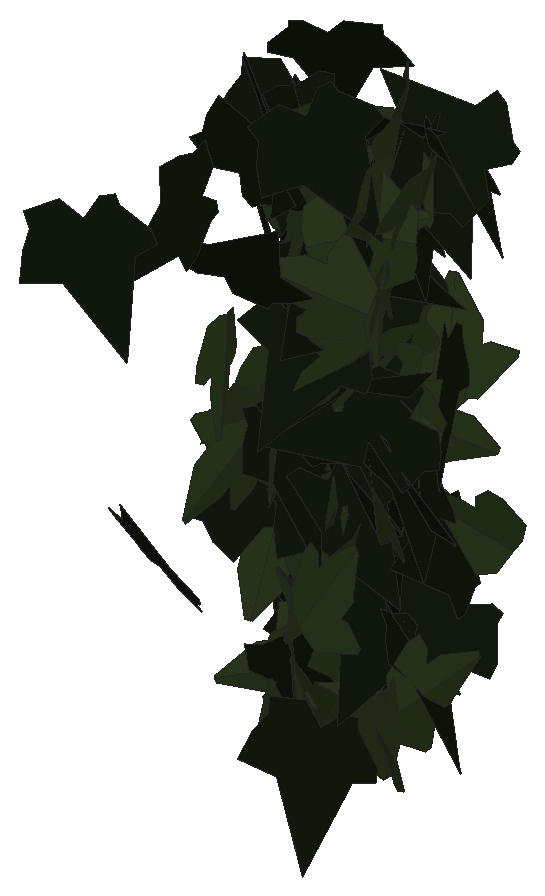
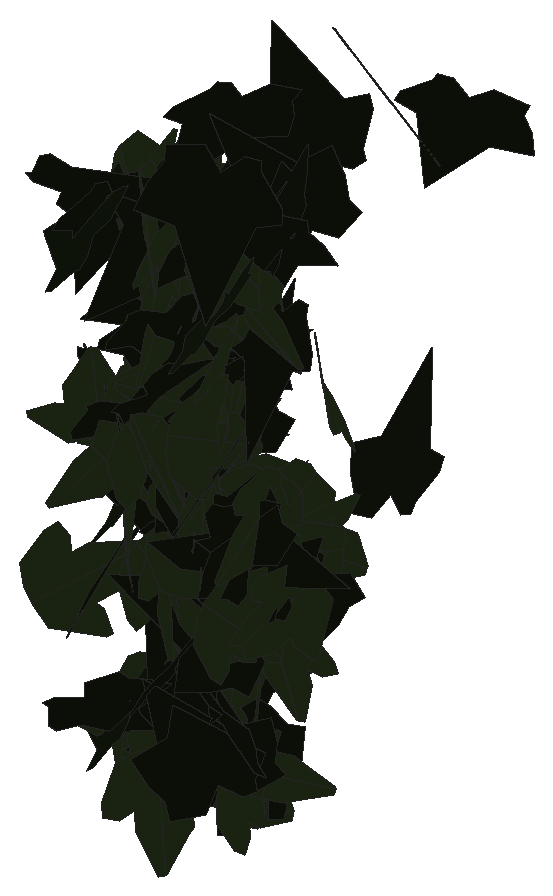
# SketchUp Ruby script. Lengths in inches.
U = 1.inch
M = Sketchup.active_model
def pt(a) = Geom::Point3d.new(a.map { |v| v * U })
def face(e, loops, mat)
  f = e.add_face(loops[0].map { |a| pt(a) })
  loops[1..].each { |l| e.add_face(l.map { |a| pt(a) }).erase! }
  f.material = f.back_material = mat if mat
  f
end
# faces: each face lists its corners as indices into pts; further lists are holes
def faces(e, pts, list, mat = nil) = list.each { |f| face(e, (f[0].is_a?(Array) ? f : [f]).map { |l| l.map { |i| pts[i] } }, mat) }
# xy, xz, yz: faces in a plane at the given z, y or x. An outline is a flat list of corners, or four numbers for a rectangle; further outlines are holes
def ring(l) = l.size == 4 ? [[l[0], l[1]], [l[2], l[1]], [l[2], l[3]], [l[0], l[3]]] : l.each_slice(2).to_a
def flat(e, list, mat, &to3) = list.each { |f| face(e, (f[0].is_a?(Array) ? f : [f]).map { |l| ring(l).map { |u, v| to3.(u, v) } }, mat) }
def xy(e, z, list, mat = nil) = flat(e, list, mat) { |x, y| [x, y, z] }
def xz(e, y, list, mat = nil) = flat(e, list, mat) { |x, z| [x, y, z] }
def yz(e, x, list, mat = nil) = flat(e, list, mat) { |y, z| [x, y, z] }
def lines(e, pts, list) = list.each { |a, b| e.add_line(pt(pts[a]), pt(pts[b])) }
# prism: a flat outline (further loops are holes) pulled along v
def prism(e, loops, v, mat = nil)
  f = face(e, loops, mat); d = Geom::Vector3d.new(v.map { |x| x * U })
  f.pushpull(f.normal.samedirection?(d) ? d.length : -d.length)
end
def box(e, o, s, mat = nil) = prism(e, [[o, [o[0] + s[0], o[1], o[2]], [o[0] + s[0], o[1] + s[1], o[2]], [o[0], o[1] + s[1], o[2]]]], [0, 0, s[2]], mat)
def at(x, y, z, deg = 0) = Geom::Transformation.translation(pt([x, y, z])) * Geom::Transformation.rotation(ORIGIN, Z_AXIS, deg.degrees)
def axes(o, x, y, z) = Geom::Transformation.new([*x, 0, *y, 0, *z, 0, *pt(o).to_a, 1])
def part(name) = M.definitions.add(name)
# library, detail: a bought-in or finely detailed component or shape, given as its bounding box
def library(name, o, s) = part(name).tap { |d| box(d.entities, o, s) }
def detail(e, o, s) = box(e.add_group.entities, o, s)
def put(e, d, t, mat = nil) = e.add_instance(d, t).tap { |i| i.material = mat if mat }
def group(e, t, mat = nil) = e.add_group.tap { |g| g.transformation = t; g.material = mat if mat }.entities
root = M.entities
M.materials.add("efeu1").color = [18, 25, 13]
M.materials.add("efeu2").color = [43, 57, 29]
c1 = part("ivyleaf_10")
p = [[0,0.5,-0.03],[-0.0625,2.02,-0.43],[-0.19,2.01,-0.46],[-0.54,1.05,-0.29],[-0.52,0.625,-0.18],[-0.83,0.76,-0.28],
  [-1.16,0.64,-0.33],[-1.15,0.33,-0.24],[-0.77,-0.39,0.02],[-0.3,-0.51,0.16],[0.04,-0.48,0.23],[-0.02,2.01,-0.4375],
  [-0.06,2.01,-0.43],[0.04,-0.49,0.23],[0.67,-0.49,0.14],[1.38,0.36,-0.2],[1.375,0.51,-0.24],[0.81,0.65,-0.19],
  [0.62,0.59,-0.15],[0.6,1.09,-0.28],[0.5,1.23,-0.31]]
faces(c1.entities,p,[[0,1,2,3,4,5,6,7,8,9,10],[11,12,0,13,14,15,16,17,18,19,20]],"efeu2")
c2 = part("ivyleaf_9")
p = [[1.54,2.16,1.25],[1.36,2.04,1.19],[-0.21,0.99,0.68],[-0.71,1.11,0.82],[-0.85,0.86,0.67],[-0.8,0.17,0.21],
  [-0.9,-0.01,0.1],[-0.67,-0.16,-0.02],[-0.08,-0.08,-0.05],[-0.03,-0.6,-0.4],[0.65,-0.88,-0.66],[0.83,-0.6,-0.49],
  [1.29,-0.42,-0.43],[1.8125,-0.07,-0.26],[1.21,0.44,0.15]]
faces(c2.entities,p,[[0,1,2,3,4,5,6,7,8,9,10,11,12,13,14]],"efeu1")
put(root,c1,axes([22.39,223.125,209.93],[-0.0897,-0.2563,0.41984],[0.06597,-0.42918,-0.2479],[0.48744,0.01092,0.11081]))
put(root,c1,axes([22.26,223.42,209.56],[-0.10098,-0.23704,-0.4285],[0.24767,0.35271,-0.25348],[0.42245,-0.26345,0.04618]))
put(root,c1,axes([22.4,223.66,210.71],[-0.06365,-0.30716,-0.38936],[0.12661,0.36948,-0.31218],[0.4795,-0.13833,0.03074]))
put(root,c2,axes([22.47,223.47,212.67],[0.39377,0.05148,-0.3038],[-0.30381,-0.0174,-0.39673],[-0.05142,0.49704,0.01758]))
put(root,c1,axes([22.43,223.16,210.55],[-0.10468,-0.28696,-0.39585],[0.18073,0.35344,-0.30401],[0.45429,-0.20673,0.02972]))
put(root,c1,axes([22.28,223.0625,209.86],[0.10985,-0.06556,-0.48336],[0.34124,0.36437,0.02813],[0.34855,-0.33606,0.12479]))
put(root,c1,axes([22.57,224.26,209.58],[-0.0425,-0.32943,0.37373],[0.0224,-0.37597,-0.32885],[0.49769,-0.01121,0.04672]))
put(root,c2,axes([22.79,224.08,210.3],[-0.03883,-0.0473,-0.49624],[-0.13963,-0.47679,0.05637],[-0.47854,0.14295,0.02382]))
put(root,c1,axes([22.86,223.45,212.68],[0.14303,-0.07475,-0.47324],[-0.39555,0.26025,-0.16066],[0.27034,0.42034,0.01531]))
put(root,c2,axes([22.38,223.03,209.57],[0.12232,-0.06453,-0.48049],[0.03974,0.49522,-0.05639],[0.48318,-0.02439,0.12628]))
put(root,c2,axes([22.41,224.34,211.38],[0.07234,-0.44625,0.2136],[0.02764,-0.21189,-0.45204],[0.49397,0.07721,-0.00599]))
put(root,c1,axes([22.6,223.1,210],[-0.01888,-0.3413,-0.36491],[0.12465,0.35041,-0.33418],[0.48385,-0.10359,0.07185]))
put(root,c2,axes([22.58,223.72,213.77],[-0.32543,-0.29744,-0.23584],[0.16978,0.1638,-0.44085],[0.33951,-0.36701,-0.00561]))
put(root,c1,axes([22.6,223.32,208.92],[0.49822,0.03064,-0.02887],[-0.02881,-0.00188,-0.49917],[-0.0307,0.49906,-0.00011]))
put(root,c2,axes([22.41,223.56,209.78],[0.07247,0.03093,0.49375],[0.44759,0.20848,-0.07876],[-0.21075,0.45341,0.00253]))
put(root,c1,axes([22.86,223.7,210.61],[0.36351,0.10917,-0.32549],[-0.31996,-0.06411,-0.37883],[-0.12446,0.4837,0.02325]))
put(root,c1,axes([22.99,223.56,207.39],[-0.0838,-0.0172,0.49263],[-0.32526,-0.37354,-0.06838],[0.37038,-0.33192,0.05142]))
put(root,c2,axes([22.46,223.42,213.62],[0.08486,-0.21763,0.44208],[0.14192,-0.41879,-0.2334],[0.47187,0.16509,-0.0093]))
put(root,c2,axes([22.8125,224,214.37],[0.29922,0.34084,-0.21046],[-0.13722,-0.15959,-0.45354],[-0.37634,0.32918,-0.00196]))
put(root,c2,axes([22.58,220.34,213.72],[-0.19688,-0.27431,-0.36877],[0.22296,0.29381,-0.33758],[0.4019,-0.29737,0.00663]))
put(root,c1,axes([22.75,223.78,207.35],[0.0185,-0.28996,0.40692],[0.0875,-0.39902,-0.28832],[0.49194,0.08188,0.03597]))
put(root,c1,axes([22.57,222.5625,211.42],[0.34049,-0.1951,0.30984],[0.26,-0.16908,-0.39219],[0.25781,0.42819,-0.01368]))
put(root,c1,axes([22.9375,223.84,213.44],[-0.08729,-0.38274,0.30967],[-0.07979,-0.29934,-0.39246],[0.48581,-0.11793,-0.00882]))
put(root,c2,axes([22.67,224.24,207.7],[0.33857,0.30926,0.19931],[-0.15139,-0.12977,0.45852],[0.33533,-0.37083,0.00577]))
put(root,c1,axes([22.89,224.37,211.54],[0.02201,-0.19577,0.45955],[0.02433,-0.45903,-0.19672],[0.49892,0.03102,-0.01067]))
put(root,c2,axes([22.48,224.03,210.16],[0.09228,-0.14945,0.46813],[0.4572,-0.14851,-0.13753],[0.18016,0.45344,0.10925]))
put(root,c1,axes([22.92,224.21,209.96],[-0.18048,-0.45016,-0.1216],[-0.0446,-0.11313,0.48499],[-0.46415,0.1859,0.00068]))
put(root,c2,axes([22.82,223.73,213.34],[-0.02864,-0.3446,0.36115],[-0.023,-0.36045,-0.34576],[0.49865,-0.03642,0.00479]))
put(root,c2,axes([22.78,224.38,210.89],[-0.00931,-0.3587,0.34821],[0.02769,-0.3481,-0.35785],[0.49915,0.01262,0.02634]))
put(root,c2,axes([22.71,223.31,211.99],[0.03728,-0.16241,0.47142],[0.10973,-0.45847,-0.16663],[0.48638,0.11588,0.00146]))
put(root,c2,axes([22.7,224.22,212.9],[0.1452,-0.43605,0.19691],[0.08286,-0.17975,-0.45916],[0.47122,0.16597,0.02006]))
put(root,c1,axes([22.85,223.45,207.92],[-0.11731,0.38912,-0.29125],[0.08213,-0.27943,-0.40641],[-0.47906,-0.14319,0.00165]))
put(root,c1,axes([22.91,223.76,212.34],[-0.17262,0.46599,-0.05528],[0.01801,-0.05228,-0.49693],[-0.46891,-0.17355,0.00126]))
put(root,c2,axes([22.61,223.88,209.22],[0.32085,0.22039,-0.31382],[0.16505,0.28997,0.37239],[0.34614,-0.34256,0.11333]))
put(root,c2,axes([22.86,223.85,207.89],[-0.28892,0.26842,0.30737],[0.22624,-0.20807,0.39436],[0.33962,0.36696,-0.00123]))
put(root,c2,axes([22.84,223.93,207.51],[-0.24358,-0.04545,0.43428],[0.43386,0.03103,0.24659],[-0.04937,0.49696,0.02432]))
put(root,c2,axes([22.91,221.14,209.55],[0.41349,-0.27632,0.05168],[-0.04286,0.02887,0.49732],[-0.27782,-0.41571,0.00019]))
put(root,c1,axes([23.26,223.63,211.26],[-0.15313,0.18048,-0.44043],[-0.26676,0.35063,0.23643],[0.3942,0.30739,-0.0111]))
put(root,c1,axes([22.8,223.29,210],[-0.01139,-0.06945,0.49502],[0.33392,-0.36952,-0.04416],[0.37198,0.32959,0.0548]))
put(root,c1,axes([23.0625,223.66,210.7],[-0.28499,-0.38138,-0.15275],[-0.09408,-0.12038,0.47609],[-0.39991,0.3001,-0.00314]))
put(root,c2,axes([22.7,222.75,213.33],[-0.04647,-0.04604,0.4957],[0.46127,-0.19127,0.02548],[0.18728,0.45967,0.06025]))
put(root,c2,axes([22.93,223.13,210.2],[0.16655,-0.47101,-0.02021],[-0.00122,0.021,-0.49956],[0.47145,0.16645,0.00584]))
put(root,c2,axes([22.81,223.24,207.24],[0.24881,0.00437,0.43368],[0.43369,-0.00578,-0.24876],[0.00284,0.49995,-0.00667]))
put(root,c1,axes([23.11,224.22,209.54],[0.46025,-0.12585,0.14942],[0.14358,-0.04142,-0.47715],[0.13248,0.48213,-0.00198]))
put(root,c2,axes([23.29,223.89,211.61],[-0.21485,-0.32933,0.30884],[-0.10358,-0.29695,-0.38871],[0.43945,-0.231,0.05938]))
put(root,c1,axes([23.6,223.12,207.93],[-0.29193,0.15126,-0.3767],[-0.35936,0.11948,0.32647],[0.18878,0.46135,0.03895]))
put(root,c1,axes([23.57,223.54,212.65],[0.25723,0.07284,-0.42252],[-0.42849,0.06118,-0.25031],[0.01523,0.49087,0.0939]))
put(root,c1,axes([23.34,223.97,209.87],[-0.11715,-0.47106,-0.1199],[0.01547,0.11966,-0.48522],[0.48584,-0.1174,-0.01347]))
put(root,c2,axes([23.14,224.34,208.875],[0.03103,-0.47058,0.16612],[0.00852,-0.16591,-0.47159],[0.49896,0.0321,-0.00228]))
put(root,c1,axes([23.44,224.2,207.45],[-0.38144,-0.31886,0.05325],[-0.04192,-0.03288,-0.49715],[0.32054,-0.38373,-0.00165]))
put(root,c1,axes([23.0625,223.25,208.84],[0.31827,-0.17464,-0.34381],[0.29953,-0.1688,0.36303],[-0.24287,-0.43704,-0.00283]))
put(root,c1,axes([23.45,223.92,213.22],[-0.16563,-0.38402,0.27403],[-0.01208,-0.28689,-0.40933],[0.47161,-0.14222,0.08576]))
put(root,c1,axes([23.57,223.53,210.57],[0.10577,-0.16027,-0.46165],[-0.21367,0.40963,-0.19117],[0.43949,0.23773,0.01817]))
put(root,c1,axes([23.03,223.92,211.63],[-0.01861,-0.06589,0.49529],[0.46027,0.19061,0.04265],[-0.19443,0.45752,0.05356]))
put(root,c2,axes([23,223.43,211.32],[0.35706,-0.2045,0.28405],[0.24738,-0.13962,-0.41147],[0.24761,0.43438,0.00147]))
put(root,c1,axes([23.53,223.12,211.5],[-0.0624,0.11918,0.48156],[-0.23572,0.41994,-0.13447],[-0.43651,-0.24381,0.00378]))
put(root,c2,axes([23.61,220.88,214.14],[-0.4689,0.15834,-0.07115],[0.06681,-0.02454,-0.49491],[-0.16022,-0.47363,0.00185]))
put(root,c2,axes([23.31,224.19,212.73],[-0.16153,-0.46076,-0.10776],[0.04036,0.10003,-0.48823],[0.47146,-0.16643,0.00488]))
put(root,c2,axes([23.36,223.36,210.86],[0.40143,0.28876,-0.07397],[-0.06239,-0.03994,-0.49448],[-0.29148,0.40623,0.00397]))
put(root,c1,axes([23.25,223.76,213.31],[-0.21561,0.23035,-0.38788],[0.21173,-0.32794,-0.31245],[-0.39835,-0.29899,0.04387]))
put(root,c2,axes([23.55,224.125,211.71],[-0.30277,-0.33517,0.21445],[-0.14574,-0.15734,-0.45167],[0.37026,-0.33601,-0.00242]))
put(root,c2,axes([23.375,223.36,211.88],[-0.12348,-0.31763,0.36588],[0.01229,-0.3795,-0.32531],[0.48436,-0.07135,0.10153]))
put(root,c1,axes([23.3125,223.74,209.64],[-0.02401,-0.02604,0.49874],[0.29476,-0.40382,-0.00689],[0.40316,0.29369,0.03474]))
put(root,c1,axes([23.49,222.76,213.08],[0.32218,-0.38068,0.03584],[0.01879,-0.03105,-0.49868],[0.3819,0.32268,-0.0057]))
put(root,c1,axes([23.47,223.11,208.6875],[-0.09937,-0.40082,-0.28191],[0.12129,0.25858,-0.4104],[0.47478,-0.14995,0.04584]))
put(root,c1,axes([23.64,224.125,211.21],[0.42802,-0.14124,-0.21644],[-0.1976,0.09106,-0.45018],[0.16659,0.47091,0.02214]))
put(root,c1,axes([23.55,223.82,212.76],[-0.0086,-0.37565,-0.32987],[0.042,0.32821,-0.37485],[0.49816,-0.03415,0.02591]))
put(root,c1,axes([23.48,223.875,213.54],[-0.01184,0.45605,-0.20464],[-0.00824,-0.20485,-0.45604],[-0.49979,-0.00743,0.01236]))
put(root,c2,axes([23.3,223.97,208.15],[-0.11592,-0.0525,0.48354],[0.29968,-0.39923,0.0285],[0.38309,0.29641,0.12402]))
put(root,c2,axes([23.59,222.99,211.73],[-0.29398,-0.39992,0.06029],[-0.0264,-0.0554,-0.49622],[0.40358,-0.29494,0.01145]))
put(root,c1,axes([23.42,223.83,212.82],[0.45662,0.1814,0.09267],[0.08725,0.03137,-0.49133],[-0.18407,0.46488,-0.003]))
put(root,c1,axes([23.42,223.97,210.75],[0.34693,-0.26632,0.24231],[0.19192,-0.14792,-0.43736],[0.30464,0.39647,-0.00041]))
put(root,c1,axes([23.69,223.59,207.25],[0.24051,0.38307,0.2131],[-0.11737,-0.17791,0.4523],[0.42235,-0.26758,0.00434]))
put(root,c1,axes([23.69,223.96,209.67],[-0.10612,-0.40905,0.26724],[-0.05898,-0.26075,-0.42253],[0.48504,-0.1212,0.00709]))
put(root,c1,axes([23.41,223.12,207.03],[-0.35301,0.09905,0.33996],[0.31895,-0.11954,0.36603],[0.15379,0.47529,0.02122]))
put(root,c2,axes([23.48,223.66,213.57],[0.41761,0.25925,0.0916],[0.07184,0.05791,-0.49141],[-0.2654,0.4236,0.01111]))
put(root,c1,axes([23.7,224.03,213.91],[0.19514,-0.43601,-0.1477],[-0.03558,0.14566,-0.47699],[0.45897,0.19667,0.02582]))
put(root,c1,axes([23.75,224.05,211.0625],[-0.13328,-0.37358,0.30443],[-0.02748,-0.30945,-0.39177],[0.48112,-0.12116,0.06195]))
put(root,c2,axes([23.3125,223.55,209.48],[0.13916,-0.15805,0.45349],[0.2759,-0.36015,-0.21018],[0.39308,0.30873,-0.01302]))
put(root,c1,axes([23.74,223.125,209.11],[0.04399,-0.48722,-0.10333],[-0.0076,0.10306,-0.4892],[0.498,0.04461,0.00166]))
put(root,c2,axes([23.52,223.13,209.8],[-0.0678,-0.30171,-0.39291],[0.11513,0.37611,-0.30868],[0.48182,-0.13233,0.01847]))
put(root,c1,axes([23.75,223.67,210.45],[0.27961,-0.38211,0.16066],[-0.09897,0.12665,0.47346],[-0.40252,-0.29657,-0.00481]))
put(root,c1,axes([23.74,223.46,212.74],[-0.36558,0.33822,-0.04424],[0.02903,-0.03375,-0.49801],[-0.33987,-0.3667,0.00504]))
put(root,c1,axes([23.88,223.11,211.46],[-0.0354,-0.26273,0.42393],[-0.07058,-0.41808,-0.265],[0.49373,-0.0786,-0.00749]))
put(root,c2,axes([23.48,222.85,210.55],[0.01517,-0.01843,0.49943],[0.49884,0.03102,-0.01401],[-0.03047,0.4987,0.01933]))
put(root,c2,axes([23.7,223.73,212.1875],[-0.23668,-0.36797,-0.24203],[0.13869,0.19851,-0.43744],[0.41803,-0.2742,0.0081]))
put(root,c1,axes([24.01,224.05,211.28],[0.05758,0.1059,-0.48525],[-0.31462,-0.37022,-0.11813],[-0.38432,0.31894,0.024]))
put(root,c2,axes([23.8125,224.17,211.51],[-0.22561,-0.43916,-0.07901],[0.03662,0.07001,-0.49372],[0.4447,-0.22856,0.00058]))
put(root,c2,axes([23.53,223.21,212.58],[0.04861,0.06363,-0.49355],[0.30493,0.38808,0.08007],[0.39326,-0.30878,-0.00108]))
put(root,c1,axes([23.94,223.75,213.41],[0.46581,-0.0855,-0.16034],[-0.15709,0.03233,-0.47358],[0.09134,0.49157,0.00326]))
put(root,c2,axes([23.6875,222.58,214.32],[0.01779,-0.34568,-0.36082],[0.06465,0.35961,-0.34133],[0.49548,-0.03451,0.05749]))
put(root,c2,axes([23.625,223.33,213.19],[0.09353,-0.35679,0.33756],[0.13038,-0.31327,-0.36724],[0.47355,0.15672,0.03443]))
put(root,c1,axes([23.75,223.47,212.57],[-0.07681,0.21672,-0.444],[0.14789,-0.41864,-0.22993],[-0.47141,-0.16665,0.00021]))
put(root,c2,axes([23.86,223.57,208.22],[-0.08129,-0.42771,0.24589],[-0.0232,-0.24561,-0.4349],[0.4928,-0.08211,0.02009]))
put(root,c2,axes([23.69,221.26,213.11],[0.48681,0.1072,-0.03907],[0.03536,0.02102,0.4983],[0.10848,-0.48792,0.01289]))
put(root,c1,axes([24.19,223.75,211.22],[0.0922,0.13918,-0.4713],[-0.28255,-0.37733,-0.1667],[-0.40207,0.29708,0.00907]))
put(root,c2,axes([24.33,223.31,210.77],[-0.07807,-0.20482,-0.4494],[-0.15714,-0.42103,0.21919],[-0.4682,0.17546,0.00137]))
put(root,c1,axes([24.45,223.02,213.02],[-0.06396,0.09235,0.48722],[-0.4646,-0.1829,-0.02632],[0.17336,-0.45609,0.10921]))
put(root,c2,axes([23.99,222.36,207.45],[-0.13828,-0.47774,-0.0514],[0.02069,0.04752,-0.49731],[0.48005,-0.13967,0.00663]))
put(root,c1,axes([24.14,223.16,207.45],[-0.16917,-0.46291,-0.08425],[0.02777,0.07955,-0.49285],[0.46969,-0.17143,-0.0012]))
put(root,c1,axes([23.95,223.59,213.61],[0.13702,-0.26304,0.40254],[0.23467,-0.32876,-0.29471],[0.41971,0.26969,0.03336]))
put(root,c1,axes([23.79,222.81,212.89],[0.13203,0.03409,-0.48105],[0.44988,0.17096,0.13559],[0.17372,-0.46863,0.01447]))
put(root,c1,axes([23.86,224.09,209.8],[0.01654,-0.04242,0.49792],[0.40735,-0.28743,-0.03802],[0.28946,0.40692,0.02505]))
put(root,c2,axes([24.22,224.31,208.11],[-0.3506,-0.34936,0.0709],[-0.04385,-0.05642,-0.49487],[0.35378,-0.35322,0.00892]))
put(root,c1,axes([24.38,222.84,210.07],[-0.33951,0.19731,0.30951],[-0.2657,0.15879,-0.39267],[-0.25325,-0.43111,-0.00297]))
put(root,c2,axes([23.92,223.83,213.01],[0.13611,-0.39452,0.27538],[0.10712,-0.25415,-0.41705],[0.46904,0.17252,0.01534]))
put(root,c1,axes([23.96,223.24,212.46],[0.33751,-0.17462,0.32496],[0.29101,-0.14466,-0.37998],[0.22672,0.44563,0.00399]))
put(root,c1,axes([24.22,222.79,213.39],[-0.02083,-0.2626,-0.42498],[0.03622,0.42343,-0.26343],[0.49825,-0.04176,0.00138]))
put(root,c1,axes([24.17,223.34,212.52],[0.18726,-0.44524,0.12921],[0.06591,-0.11237,-0.48273],[0.4589,0.19783,0.01661]))
put(root,c2,axes([23.81,223.41,210.1],[0.16179,0.04816,-0.47064],[0.46166,0.09265,0.16818],[0.1034,-0.48898,-0.01448]))
put(root,c1,axes([23.875,223.45,211.04],[0.21642,0.05533,0.44733],[0.42089,0.15275,-0.22253],[-0.16129,0.47287,0.01954]))
put(root,c1,axes([24.55,222.07,212.74],[0.13398,0.09405,0.47245],[-0.39276,-0.2626,0.16365],[0.27891,-0.41496,0.00351]))
put(root,c2,axes([24.16,223.85,213.65],[0.00404,-0.41042,-0.28554],[-0.01791,0.28525,-0.41026],[0.49966,0.01354,-0.0124]))
put(root,c1,axes([24.08,222.16,208.99],[0.39748,-0.15179,-0.26263],[0.24297,-0.09986,0.42543],[-0.1816,-0.46582,-0.00562]))
put(root,c2,axes([24.06,223.84,207.83],[0.23393,-0.42271,0.12883],[0.06192,-0.11298,-0.48312],[0.43754,0.24198,-0.00051]))
put(root,c2,axes([24.74,224.01,213.54],[-0.40534,-0.19382,-0.21938],[-0.19894,-0.09251,0.4493],[-0.21476,0.45153,-0.00212]))
put(root,c1,axes([24.34,223.99,211.05],[0.40741,0.2856,-0.04949],[0.03047,0.04269,0.49724],[0.28825,-0.40818,0.01738]))
put(root,c1,axes([24.73,224.21,209.13],[-0.24674,-0.07692,-0.42802],[-0.40775,-0.13017,0.25845],[-0.15119,0.47659,0.00151]))
put(root,c1,axes([24.74,222.64,207.4],[-0.01399,0.00892,0.49972],[-0.45939,0.19671,-0.01637],[-0.19689,-0.45959,0.00269]))
put(root,c2,axes([24.125,224.39,213.44],[0.21929,-0.40128,0.2022],[0.11879,-0.16522,-0.45672],[0.43336,0.24835,0.02287]))
put(root,c2,axes([24.22,223.5625,210.11],[0.09925,-0.44389,0.20763],[0.07498,-0.19559,-0.45401],[0.48428,0.12126,0.02775]))
put(root,c1,axes([24.33,223.54,210.67],[-0.15025,-0.24813,-0.40725],[0.28081,0.29908,-0.28583],[0.38545,-0.31461,0.04948]))
put(root,c2,axes([24.45,224.04,209],[-0.12633,-0.14982,0.45999],[-0.08122,-0.4621,-0.17281],[0.47691,-0.11838,0.09242]))
put(root,c1,axes([24.53,223.27,213.54],[0.10935,-0.48689,0.03131],[0.00949,-0.02996,-0.49901],[0.4878,0.10973,0.00269]))
put(root,c1,axes([24.45,223.21,207.6],[0.05003,0.0386,-0.49599],[0.16208,0.47003,0.05293],[0.47035,-0.16608,0.03452]))
put(root,c2,axes([24.41,223.9,211.4],[-0.29249,0.0308,-0.40435],[0.40433,-0.01604,-0.2937],[-0.03106,-0.49879,-0.01552]))
